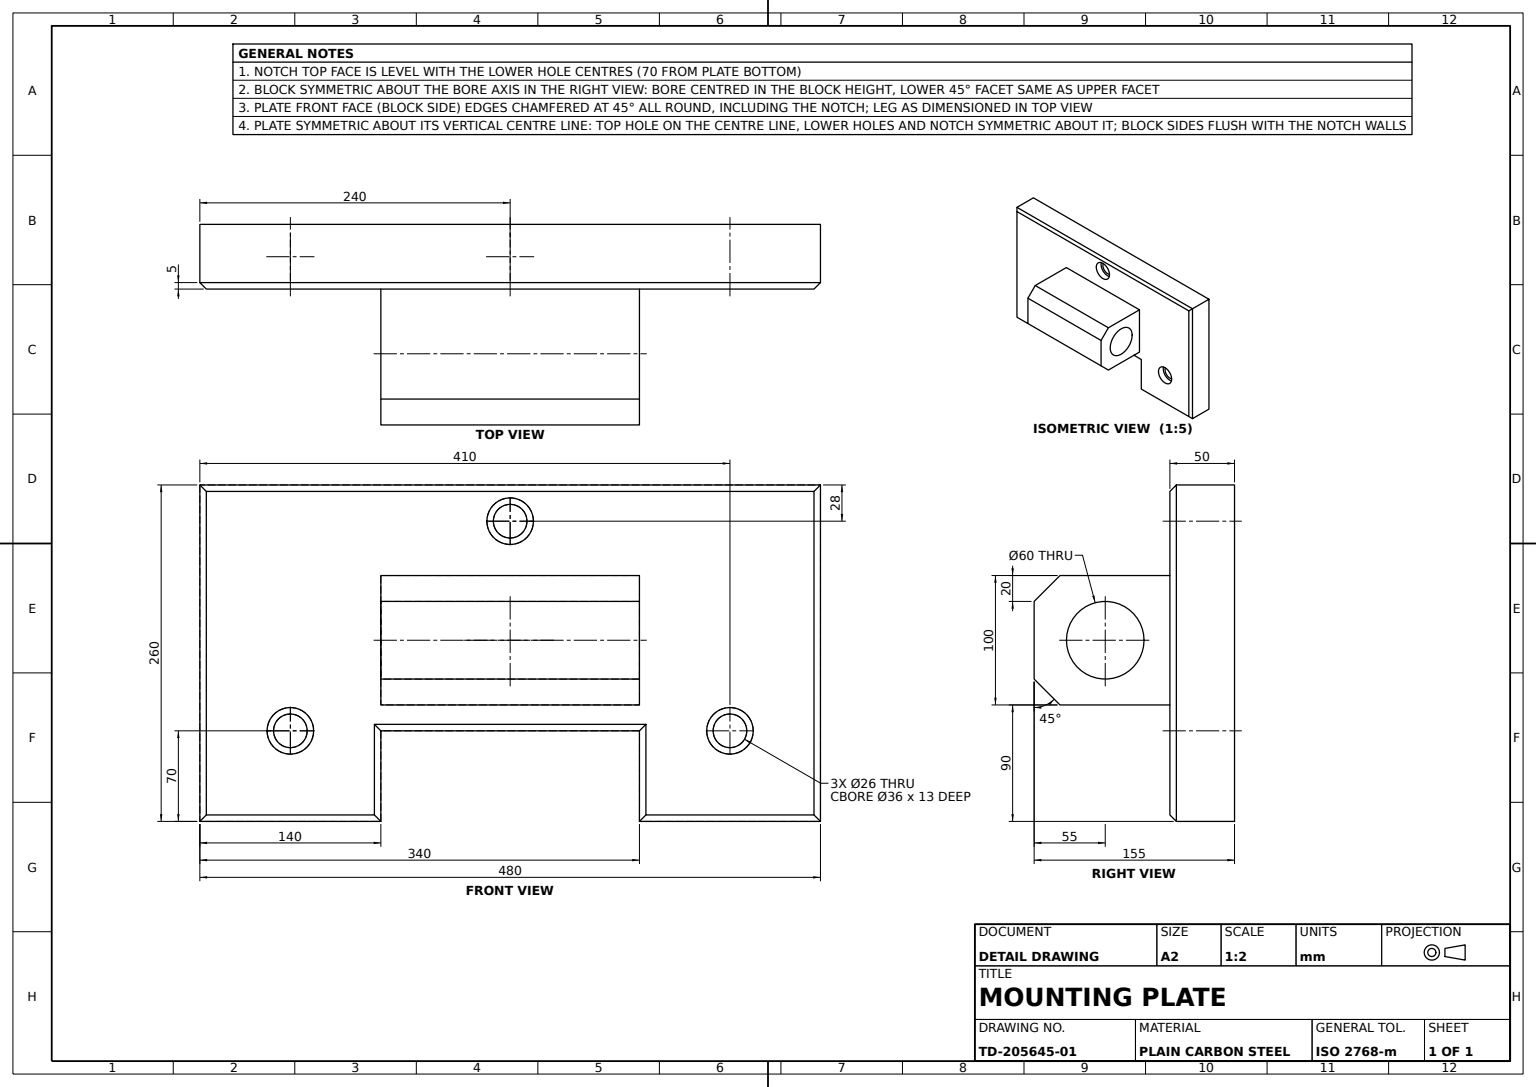
ISO-10303-21;
HEADER;
FILE_DESCRIPTION((''),'2;1');
FILE_NAME('','',(''),(''),'','','');
FILE_SCHEMA(('AUTOMOTIVE_DESIGN'));
ENDSEC;
DATA;
#1=APPLICATION_CONTEXT('');
#2=PRODUCT_CONTEXT('',#1,'mechanical');
#3=PRODUCT('','','',(#2));
#4=PRODUCT_DEFINITION_FORMATION('','',#3);
#5=PRODUCT_DEFINITION_CONTEXT('',#1,'design');
#6=PRODUCT_DEFINITION('','',#4,#5);
#7=PRODUCT_DEFINITION_SHAPE('','',#6);
#8=(LENGTH_UNIT()NAMED_UNIT(*)SI_UNIT(.MILLI.,.METRE.));
#9=(NAMED_UNIT(*)PLANE_ANGLE_UNIT()SI_UNIT($,.RADIAN.));
#10=(NAMED_UNIT(*)SI_UNIT($,.STERADIAN.)SOLID_ANGLE_UNIT());
#11=UNCERTAINTY_MEASURE_WITH_UNIT(LENGTH_MEASURE(1.E-05),#8,'distance_accuracy_value','');
#12=(GEOMETRIC_REPRESENTATION_CONTEXT(3)GLOBAL_UNCERTAINTY_ASSIGNED_CONTEXT((#11))GLOBAL_UNIT_ASSIGNED_CONTEXT((#8,#9,#10))REPRESENTATION_CONTEXT('',''));
#13=CARTESIAN_POINT('',(428.,-190.,37.));
#14=VERTEX_POINT('',#13);
#15=CARTESIAN_POINT('',(428.,-190.,50.));
#16=VERTEX_POINT('',#15);
#17=DIRECTION('',(0.,0.,1.));
#18=VECTOR('',#17,1000.);
#19=LINE('',#13,#18);
#20=EDGE_CURVE('',#14,#16,#19,.T.);
#21=ORIENTED_EDGE('',*,*,#20,.T.);
#22=CARTESIAN_POINT('',(392.,-190.,50.));
#23=VERTEX_POINT('',#22);
#24=CARTESIAN_POINT('',(410.,-190.,50.));
#25=DIRECTION('',(1.,0.,0.));
#26=AXIS2_PLACEMENT_3D('',#24,#17,#25);
#27=CIRCLE('',#26,18.);
#28=EDGE_CURVE('',#16,#23,#27,.T.);
#29=ORIENTED_EDGE('',*,*,#28,.T.);
#30=CARTESIAN_POINT('',(392.,-190.,37.));
#31=VERTEX_POINT('',#30);
#32=LINE('',#30,#18);
#33=EDGE_CURVE('',#31,#23,#32,.T.);
#34=ORIENTED_EDGE('',*,*,#33,.F.);
#35=CARTESIAN_POINT('',(410.,-190.,37.));
#36=AXIS2_PLACEMENT_3D('',#35,#17,#25);
#37=CIRCLE('',#36,18.);
#38=EDGE_CURVE('',#14,#31,#37,.T.);
#39=ORIENTED_EDGE('',*,*,#38,.F.);
#40=EDGE_LOOP('',(#21,#29,#34,#39));
#41=FACE_OUTER_BOUND('',#40,.T.);
#42=CYLINDRICAL_SURFACE('',#36,18.);
#43=ADVANCED_FACE('',(#41),#42,.F.);
#44=CARTESIAN_POINT('',(0.,-260.,45.));
#45=VERTEX_POINT('',#44);
#46=CARTESIAN_POINT('',(5.,-255.,50.));
#47=VERTEX_POINT('',#46);
#48=CARTESIAN_POINT('',(90.,-170.,135.));
#49=DIRECTION('',(0.577350269,0.577350269,0.577350269));
#50=VECTOR('',#49,1000.);
#51=LINE('',#48,#50);
#52=EDGE_CURVE('',#45,#47,#51,.T.);
#53=ORIENTED_EDGE('',*,*,#52,.F.);
#54=CARTESIAN_POINT('',(140.,-260.,45.));
#55=VERTEX_POINT('',#54);
#56=DIRECTION('',(-1.,0.,0.));
#57=VECTOR('',#56,1000.);
#58=LINE('',#54,#57);
#59=EDGE_CURVE('',#55,#45,#58,.T.);
#60=ORIENTED_EDGE('',*,*,#59,.F.);
#61=CARTESIAN_POINT('',(135.,-255.,50.));
#62=VERTEX_POINT('',#61);
#63=CARTESIAN_POINT('',(90.,-210.,95.));
#64=DIRECTION('',(-0.577350269,0.577350269,0.577350269));
#65=VECTOR('',#64,1000.);
#66=LINE('',#63,#65);
#67=EDGE_CURVE('',#55,#62,#66,.T.);
#68=ORIENTED_EDGE('',*,*,#67,.T.);
#69=CARTESIAN_POINT('',(0.,-255.,50.));
#70=VECTOR('',#25,1000.);
#71=LINE('',#69,#70);
#72=EDGE_CURVE('',#47,#62,#71,.T.);
#73=ORIENTED_EDGE('',*,*,#72,.F.);
#74=EDGE_LOOP('',(#53,#60,#68,#73));
#75=FACE_OUTER_BOUND('',#74,.T.);
#76=DIRECTION('',(0.,0.707106781,-0.707106781));
#77=AXIS2_PLACEMENT_3D('',#69,#76,#25);
#78=PLANE('',#77);
#79=ADVANCED_FACE('',(#75),#78,.F.);
#80=CARTESIAN_POINT('',(340.,-90.,155.));
#81=VERTEX_POINT('',#80);
#82=CARTESIAN_POINT('',(140.,-90.,155.));
#83=VERTEX_POINT('',#82);
#84=LINE('',#80,#57);
#85=EDGE_CURVE('',#81,#83,#84,.T.);
#86=ORIENTED_EDGE('',*,*,#85,.F.);
#87=CARTESIAN_POINT('',(340.,-70.,135.));
#88=VERTEX_POINT('',#87);
#89=VECTOR('',#76,1000.);
#90=LINE('',#80,#89);
#91=EDGE_CURVE('',#81,#88,#90,.T.);
#92=ORIENTED_EDGE('',*,*,#91,.T.);
#93=CARTESIAN_POINT('',(140.,-70.,135.));
#94=VERTEX_POINT('',#93);
#95=LINE('',#87,#70);
#96=EDGE_CURVE('',#94,#88,#95,.T.);
#97=ORIENTED_EDGE('',*,*,#96,.F.);
#98=LINE('',#82,#89);
#99=EDGE_CURVE('',#83,#94,#98,.T.);
#100=ORIENTED_EDGE('',*,*,#99,.F.);
#101=EDGE_LOOP('',(#86,#92,#97,#100));
#102=FACE_OUTER_BOUND('',#101,.T.);
#103=DIRECTION('',(0.,0.707106781,0.707106781));
#104=DIRECTION('',(0.,-0.707106781,0.707106781));
#105=AXIS2_PLACEMENT_3D('',#80,#103,#104);
#106=PLANE('',#105);
#107=ADVANCED_FACE('',(#102),#106,.T.);
#108=CARTESIAN_POINT('',(57.,-190.,0.));
#109=VERTEX_POINT('',#108);
#110=CARTESIAN_POINT('',(57.,-190.,37.));
#111=VERTEX_POINT('',#110);
#112=CARTESIAN_POINT('',(57.,-190.,-19.));
#113=LINE('',#112,#18);
#114=EDGE_CURVE('',#109,#111,#113,.T.);
#115=ORIENTED_EDGE('',*,*,#114,.F.);
#116=CARTESIAN_POINT('',(83.,-190.,0.));
#117=VERTEX_POINT('',#116);
#118=CARTESIAN_POINT('',(70.,-190.,0.));
#119=DIRECTION('',(0.,0.,-1.));
#120=AXIS2_PLACEMENT_3D('',#118,#119,#56);
#121=CIRCLE('',#120,13.);
#122=EDGE_CURVE('',#109,#117,#121,.T.);
#123=ORIENTED_EDGE('',*,*,#122,.T.);
#124=CARTESIAN_POINT('',(83.,-190.,37.));
#125=VERTEX_POINT('',#124);
#126=CARTESIAN_POINT('',(83.,-190.,-19.));
#127=LINE('',#126,#18);
#128=EDGE_CURVE('',#117,#125,#127,.T.);
#129=ORIENTED_EDGE('',*,*,#128,.T.);
#130=CARTESIAN_POINT('',(70.,-190.,37.));
#131=AXIS2_PLACEMENT_3D('',#130,#17,#25);
#132=CIRCLE('',#131,13.);
#133=EDGE_CURVE('',#125,#111,#132,.T.);
#134=ORIENTED_EDGE('',*,*,#133,.T.);
#135=EDGE_LOOP('',(#115,#123,#129,#134));
#136=FACE_OUTER_BOUND('',#135,.T.);
#137=CARTESIAN_POINT('',(70.,-190.,-19.));
#138=AXIS2_PLACEMENT_3D('',#137,#17,#25);
#139=CYLINDRICAL_SURFACE('',#138,13.);
#140=ADVANCED_FACE('',(#136),#139,.F.);
#141=CARTESIAN_POINT('',(140.,-120.,70.));
#142=VERTEX_POINT('',#141);
#143=CARTESIAN_POINT('',(140.,-120.,130.));
#144=VERTEX_POINT('',#143);
#145=CARTESIAN_POINT('',(140.,-120.,100.));
#146=AXIS2_PLACEMENT_3D('',#145,#56,#17);
#147=CIRCLE('',#146,30.);
#148=EDGE_CURVE('',#142,#144,#147,.T.);
#149=ORIENTED_EDGE('',*,*,#148,.F.);
#150=EDGE_CURVE('',#144,#142,#147,.T.);
#151=ORIENTED_EDGE('',*,*,#150,.F.);
#152=EDGE_LOOP('',(#149,#151));
#153=FACE_BOUND('',#152,.T.);
#154=CARTESIAN_POINT('',(140.,-170.,135.));
#155=VERTEX_POINT('',#154);
#156=CARTESIAN_POINT('',(140.,-150.,155.));
#157=VERTEX_POINT('',#156);
#158=VECTOR('',#103,1000.);
#159=LINE('',#156,#158);
#160=EDGE_CURVE('',#155,#157,#159,.T.);
#161=ORIENTED_EDGE('',*,*,#160,.T.);
#162=DIRECTION('',(0.,1.,0.));
#163=VECTOR('',#162,1000.);
#164=LINE('',#156,#163);
#165=EDGE_CURVE('',#157,#83,#164,.T.);
#166=ORIENTED_EDGE('',*,*,#165,.T.);
#167=ORIENTED_EDGE('',*,*,#99,.T.);
#168=CARTESIAN_POINT('',(140.,-70.,50.));
#169=VERTEX_POINT('',#168);
#170=LINE('',#93,#18);
#171=EDGE_CURVE('',#169,#94,#170,.T.);
#172=ORIENTED_EDGE('',*,*,#171,.F.);
#173=CARTESIAN_POINT('',(140.,-170.,50.));
#174=VERTEX_POINT('',#173);
#175=CARTESIAN_POINT('',(140.,0.,50.));
#176=LINE('',#175,#163);
#177=EDGE_CURVE('',#174,#169,#176,.T.);
#178=ORIENTED_EDGE('',*,*,#177,.F.);
#179=VECTOR('',#119,1000.);
#180=LINE('',#173,#179);
#181=EDGE_CURVE('',#155,#174,#180,.T.);
#182=ORIENTED_EDGE('',*,*,#181,.F.);
#183=EDGE_LOOP('',(#161,#166,#167,#172,#178,#182));
#184=FACE_OUTER_BOUND('',#183,.T.);
#185=CARTESIAN_POINT('',(140.,0.,170.));
#186=AXIS2_PLACEMENT_3D('',#185,#56,#17);
#187=PLANE('',#186);
#188=ADVANCED_FACE('',(#153,#184),#187,.T.);
#189=CARTESIAN_POINT('',(475.,-255.,50.));
#190=VERTEX_POINT('',#189);
#191=CARTESIAN_POINT('',(480.,-260.,45.));
#192=VERTEX_POINT('',#191);
#193=CARTESIAN_POINT('',(390.,-170.,135.));
#194=DIRECTION('',(0.577350269,-0.577350269,-0.577350269));
#195=VECTOR('',#194,1000.);
#196=LINE('',#193,#195);
#197=EDGE_CURVE('',#190,#192,#196,.T.);
#198=ORIENTED_EDGE('',*,*,#197,.T.);
#199=CARTESIAN_POINT('',(480.,0.,45.));
#200=VERTEX_POINT('',#199);
#201=DIRECTION('',(0.,-1.,0.));
#202=VECTOR('',#201,1000.);
#203=LINE('',#199,#202);
#204=EDGE_CURVE('',#200,#192,#203,.T.);
#205=ORIENTED_EDGE('',*,*,#204,.F.);
#206=CARTESIAN_POINT('',(475.,-5.,50.));
#207=VERTEX_POINT('',#206);
#208=CARTESIAN_POINT('',(316.666667,-163.333333,208.333333));
#209=DIRECTION('',(0.577350269,0.577350269,-0.577350269));
#210=VECTOR('',#209,1000.);
#211=LINE('',#208,#210);
#212=EDGE_CURVE('',#207,#200,#211,.T.);
#213=ORIENTED_EDGE('',*,*,#212,.F.);
#214=CARTESIAN_POINT('',(475.,0.,50.));
#215=LINE('',#214,#163);
#216=EDGE_CURVE('',#190,#207,#215,.T.);
#217=ORIENTED_EDGE('',*,*,#216,.F.);
#218=EDGE_LOOP('',(#198,#205,#213,#217));
#219=FACE_OUTER_BOUND('',#218,.T.);
#220=DIRECTION('',(-0.707106781,0.,-0.707106781));
#221=AXIS2_PLACEMENT_3D('',#214,#220,#162);
#222=PLANE('',#221);
#223=ADVANCED_FACE('',(#219),#222,.F.);
#224=CARTESIAN_POINT('',(140.,-190.,45.));
#225=VERTEX_POINT('',#224);
#226=CARTESIAN_POINT('',(140.,-190.,0.));
#227=VERTEX_POINT('',#226);
#228=CARTESIAN_POINT('',(140.,-190.,50.));
#229=LINE('',#228,#179);
#230=EDGE_CURVE('',#225,#227,#229,.T.);
#231=ORIENTED_EDGE('',*,*,#230,.F.);
#232=LINE('',#224,#202);
#233=EDGE_CURVE('',#225,#55,#232,.T.);
#234=ORIENTED_EDGE('',*,*,#233,.T.);
#235=CARTESIAN_POINT('',(140.,-260.,0.));
#236=VERTEX_POINT('',#235);
#237=CARTESIAN_POINT('',(140.,-260.,50.));
#238=LINE('',#237,#179);
#239=EDGE_CURVE('',#55,#236,#238,.T.);
#240=ORIENTED_EDGE('',*,*,#239,.T.);
#241=LINE('',#226,#163);
#242=EDGE_CURVE('',#236,#227,#241,.T.);
#243=ORIENTED_EDGE('',*,*,#242,.T.);
#244=EDGE_LOOP('',(#231,#234,#240,#243));
#245=FACE_OUTER_BOUND('',#244,.T.);
#246=AXIS2_PLACEMENT_3D('',#228,#56,#17);
#247=PLANE('',#246);
#248=ADVANCED_FACE('',(#245),#247,.F.);
#249=ORIENTED_EDGE('',*,*,#160,.F.);
#250=CARTESIAN_POINT('',(340.,-170.,135.));
#251=VERTEX_POINT('',#250);
#252=LINE('',#154,#57);
#253=EDGE_CURVE('',#251,#155,#252,.T.);
#254=ORIENTED_EDGE('',*,*,#253,.F.);
#255=CARTESIAN_POINT('',(340.,-150.,155.));
#256=VERTEX_POINT('',#255);
#257=LINE('',#255,#158);
#258=EDGE_CURVE('',#251,#256,#257,.T.);
#259=ORIENTED_EDGE('',*,*,#258,.T.);
#260=LINE('',#255,#57);
#261=EDGE_CURVE('',#256,#157,#260,.T.);
#262=ORIENTED_EDGE('',*,*,#261,.T.);
#263=EDGE_LOOP('',(#249,#254,#259,#262));
#264=FACE_OUTER_BOUND('',#263,.T.);
#265=DIRECTION('',(0.,-0.707106781,-0.707106781));
#266=AXIS2_PLACEMENT_3D('',#255,#104,#265);
#267=PLANE('',#266);
#268=ADVANCED_FACE('',(#264),#267,.T.);
#269=CARTESIAN_POINT('',(52.,-190.,50.));
#270=VERTEX_POINT('',#269);
#271=CARTESIAN_POINT('',(88.,-190.,50.));
#272=VERTEX_POINT('',#271);
#273=CARTESIAN_POINT('',(70.,-190.,50.));
#274=AXIS2_PLACEMENT_3D('',#273,#17,#25);
#275=CIRCLE('',#274,18.);
#276=EDGE_CURVE('',#270,#272,#275,.T.);
#277=ORIENTED_EDGE('',*,*,#276,.T.);
#278=CARTESIAN_POINT('',(88.,-190.,37.));
#279=VERTEX_POINT('',#278);
#280=LINE('',#278,#18);
#281=EDGE_CURVE('',#279,#272,#280,.T.);
#282=ORIENTED_EDGE('',*,*,#281,.F.);
#283=CARTESIAN_POINT('',(52.,-190.,37.));
#284=VERTEX_POINT('',#283);
#285=CIRCLE('',#131,18.);
#286=EDGE_CURVE('',#284,#279,#285,.T.);
#287=ORIENTED_EDGE('',*,*,#286,.F.);
#288=LINE('',#283,#18);
#289=EDGE_CURVE('',#284,#270,#288,.T.);
#290=ORIENTED_EDGE('',*,*,#289,.T.);
#291=EDGE_LOOP('',(#277,#282,#287,#290));
#292=FACE_OUTER_BOUND('',#291,.T.);
#293=CYLINDRICAL_SURFACE('',#131,18.);
#294=ADVANCED_FACE('',(#292),#293,.F.);
#295=ORIENTED_EDGE('',*,*,#52,.T.);
#296=CARTESIAN_POINT('',(5.,-5.,50.));
#297=VERTEX_POINT('',#296);
#298=CARTESIAN_POINT('',(5.,0.,50.));
#299=LINE('',#298,#202);
#300=EDGE_CURVE('',#297,#47,#299,.T.);
#301=ORIENTED_EDGE('',*,*,#300,.F.);
#302=CARTESIAN_POINT('',(0.,0.,45.));
#303=VERTEX_POINT('',#302);
#304=CARTESIAN_POINT('',(3.333333,-3.333333,48.333333));
#305=DIRECTION('',(0.577350269,-0.577350269,0.577350269));
#306=VECTOR('',#305,1000.);
#307=LINE('',#304,#306);
#308=EDGE_CURVE('',#303,#297,#307,.T.);
#309=ORIENTED_EDGE('',*,*,#308,.F.);
#310=LINE('',#44,#163);
#311=EDGE_CURVE('',#45,#303,#310,.T.);
#312=ORIENTED_EDGE('',*,*,#311,.F.);
#313=EDGE_LOOP('',(#295,#301,#309,#312));
#314=FACE_OUTER_BOUND('',#313,.T.);
#315=DIRECTION('',(0.707106781,0.,-0.707106781));
#316=AXIS2_PLACEMENT_3D('',#298,#315,#201);
#317=PLANE('',#316);
#318=ADVANCED_FACE('',(#314),#317,.F.);
#319=ORIENTED_EDGE('',*,*,#233,.F.);
#320=CARTESIAN_POINT('',(135.,-185.,50.));
#321=VERTEX_POINT('',#320);
#322=CARTESIAN_POINT('',(73.333333,-123.333333,111.666667));
#323=LINE('',#322,#195);
#324=EDGE_CURVE('',#321,#225,#323,.T.);
#325=ORIENTED_EDGE('',*,*,#324,.F.);
#326=CARTESIAN_POINT('',(135.,0.,50.));
#327=LINE('',#326,#163);
#328=EDGE_CURVE('',#62,#321,#327,.T.);
#329=ORIENTED_EDGE('',*,*,#328,.F.);
#330=ORIENTED_EDGE('',*,*,#67,.F.);
#331=EDGE_LOOP('',(#319,#325,#329,#330));
#332=FACE_OUTER_BOUND('',#331,.T.);
#333=AXIS2_PLACEMENT_3D('',#326,#220,#162);
#334=PLANE('',#333);
#335=ADVANCED_FACE('',(#332),#334,.F.);
#336=CARTESIAN_POINT('',(397.,-190.,37.));
#337=VERTEX_POINT('',#336);
#338=CARTESIAN_POINT('',(423.,-190.,37.));
#339=VERTEX_POINT('',#338);
#340=CIRCLE('',#36,13.);
#341=EDGE_CURVE('',#337,#339,#340,.T.);
#342=ORIENTED_EDGE('',*,*,#341,.F.);
#343=EDGE_CURVE('',#339,#337,#340,.T.);
#344=ORIENTED_EDGE('',*,*,#343,.F.);
#345=EDGE_LOOP('',(#342,#344));
#346=FACE_BOUND('',#345,.T.);
#347=ORIENTED_EDGE('',*,*,#38,.T.);
#348=EDGE_CURVE('',#31,#14,#37,.T.);
#349=ORIENTED_EDGE('',*,*,#348,.T.);
#350=EDGE_LOOP('',(#347,#349));
#351=FACE_OUTER_BOUND('',#350,.T.);
#352=PLANE('',#36);
#353=ADVANCED_FACE('',(#346,#351),#352,.T.);
#354=CARTESIAN_POINT('',(258.,-28.,37.));
#355=VERTEX_POINT('',#354);
#356=CARTESIAN_POINT('',(222.,-28.,37.));
#357=VERTEX_POINT('',#356);
#358=CARTESIAN_POINT('',(240.,-28.,37.));
#359=AXIS2_PLACEMENT_3D('',#358,#17,#25);
#360=CIRCLE('',#359,18.);
#361=EDGE_CURVE('',#355,#357,#360,.T.);
#362=ORIENTED_EDGE('',*,*,#361,.T.);
#363=EDGE_CURVE('',#357,#355,#360,.T.);
#364=ORIENTED_EDGE('',*,*,#363,.T.);
#365=EDGE_LOOP('',(#362,#364));
#366=FACE_OUTER_BOUND('',#365,.T.);
#367=CARTESIAN_POINT('',(253.,-28.,37.));
#368=VERTEX_POINT('',#367);
#369=CARTESIAN_POINT('',(227.,-28.,37.));
#370=VERTEX_POINT('',#369);
#371=CIRCLE('',#359,13.);
#372=EDGE_CURVE('',#368,#370,#371,.T.);
#373=ORIENTED_EDGE('',*,*,#372,.F.);
#374=EDGE_CURVE('',#370,#368,#371,.T.);
#375=ORIENTED_EDGE('',*,*,#374,.F.);
#376=EDGE_LOOP('',(#373,#375));
#377=FACE_BOUND('',#376,.T.);
#378=PLANE('',#359);
#379=ADVANCED_FACE('',(#366,#377),#378,.T.);
#380=EDGE_CURVE('',#279,#284,#285,.T.);
#381=ORIENTED_EDGE('',*,*,#380,.F.);
#382=ORIENTED_EDGE('',*,*,#281,.T.);
#383=EDGE_CURVE('',#272,#270,#275,.T.);
#384=ORIENTED_EDGE('',*,*,#383,.T.);
#385=ORIENTED_EDGE('',*,*,#289,.F.);
#386=EDGE_LOOP('',(#381,#382,#384,#385));
#387=FACE_OUTER_BOUND('',#386,.T.);
#388=ADVANCED_FACE('',(#387),#293,.F.);
#389=EDGE_CURVE('',#23,#16,#27,.T.);
#390=ORIENTED_EDGE('',*,*,#389,.T.);
#391=ORIENTED_EDGE('',*,*,#20,.F.);
#392=ORIENTED_EDGE('',*,*,#348,.F.);
#393=ORIENTED_EDGE('',*,*,#33,.T.);
#394=EDGE_LOOP('',(#390,#391,#392,#393));
#395=FACE_OUTER_BOUND('',#394,.T.);
#396=ADVANCED_FACE('',(#395),#42,.F.);
#397=CARTESIAN_POINT('',(397.,-190.,0.));
#398=VERTEX_POINT('',#397);
#399=CARTESIAN_POINT('',(397.,-190.,-19.));
#400=LINE('',#399,#18);
#401=EDGE_CURVE('',#398,#337,#400,.T.);
#402=ORIENTED_EDGE('',*,*,#401,.F.);
#403=CARTESIAN_POINT('',(423.,-190.,0.));
#404=VERTEX_POINT('',#403);
#405=CARTESIAN_POINT('',(410.,-190.,0.));
#406=AXIS2_PLACEMENT_3D('',#405,#119,#56);
#407=CIRCLE('',#406,13.);
#408=EDGE_CURVE('',#398,#404,#407,.T.);
#409=ORIENTED_EDGE('',*,*,#408,.T.);
#410=CARTESIAN_POINT('',(423.,-190.,-19.));
#411=LINE('',#410,#18);
#412=EDGE_CURVE('',#404,#339,#411,.T.);
#413=ORIENTED_EDGE('',*,*,#412,.T.);
#414=ORIENTED_EDGE('',*,*,#343,.T.);
#415=EDGE_LOOP('',(#402,#409,#413,#414));
#416=FACE_OUTER_BOUND('',#415,.T.);
#417=CARTESIAN_POINT('',(410.,-190.,-19.));
#418=AXIS2_PLACEMENT_3D('',#417,#17,#25);
#419=CYLINDRICAL_SURFACE('',#418,13.);
#420=ADVANCED_FACE('',(#416),#419,.F.);
#421=CARTESIAN_POINT('',(222.,-28.,50.));
#422=VERTEX_POINT('',#421);
#423=LINE('',#356,#18);
#424=EDGE_CURVE('',#357,#422,#423,.T.);
#425=ORIENTED_EDGE('',*,*,#424,.F.);
#426=ORIENTED_EDGE('',*,*,#361,.F.);
#427=CARTESIAN_POINT('',(258.,-28.,50.));
#428=VERTEX_POINT('',#427);
#429=LINE('',#354,#18);
#430=EDGE_CURVE('',#355,#428,#429,.T.);
#431=ORIENTED_EDGE('',*,*,#430,.T.);
#432=CARTESIAN_POINT('',(240.,-28.,50.));
#433=AXIS2_PLACEMENT_3D('',#432,#17,#25);
#434=CIRCLE('',#433,18.);
#435=EDGE_CURVE('',#428,#422,#434,.T.);
#436=ORIENTED_EDGE('',*,*,#435,.T.);
#437=EDGE_LOOP('',(#425,#426,#431,#436));
#438=FACE_OUTER_BOUND('',#437,.T.);
#439=CYLINDRICAL_SURFACE('',#359,18.);
#440=ADVANCED_FACE('',(#438),#439,.F.);
#441=ORIENTED_EDGE('',*,*,#372,.T.);
#442=CARTESIAN_POINT('',(227.,-28.,0.));
#443=VERTEX_POINT('',#442);
#444=CARTESIAN_POINT('',(227.,-28.,-19.));
#445=LINE('',#444,#18);
#446=EDGE_CURVE('',#443,#370,#445,.T.);
#447=ORIENTED_EDGE('',*,*,#446,.F.);
#448=CARTESIAN_POINT('',(253.,-28.,0.));
#449=VERTEX_POINT('',#448);
#450=CARTESIAN_POINT('',(240.,-28.,0.));
#451=AXIS2_PLACEMENT_3D('',#450,#119,#56);
#452=CIRCLE('',#451,13.);
#453=EDGE_CURVE('',#443,#449,#452,.T.);
#454=ORIENTED_EDGE('',*,*,#453,.T.);
#455=CARTESIAN_POINT('',(253.,-28.,-19.));
#456=LINE('',#455,#18);
#457=EDGE_CURVE('',#449,#368,#456,.T.);
#458=ORIENTED_EDGE('',*,*,#457,.T.);
#459=EDGE_LOOP('',(#441,#447,#454,#458));
#460=FACE_OUTER_BOUND('',#459,.T.);
#461=CARTESIAN_POINT('',(240.,-28.,-19.));
#462=AXIS2_PLACEMENT_3D('',#461,#17,#25);
#463=CYLINDRICAL_SURFACE('',#462,13.);
#464=ADVANCED_FACE('',(#460),#463,.F.);
#465=ORIENTED_EDGE('',*,*,#308,.T.);
#466=CARTESIAN_POINT('',(0.,-5.,50.));
#467=LINE('',#466,#57);
#468=EDGE_CURVE('',#207,#297,#467,.T.);
#469=ORIENTED_EDGE('',*,*,#468,.F.);
#470=ORIENTED_EDGE('',*,*,#212,.T.);
#471=LINE('',#302,#70);
#472=EDGE_CURVE('',#303,#200,#471,.T.);
#473=ORIENTED_EDGE('',*,*,#472,.F.);
#474=EDGE_LOOP('',(#465,#469,#470,#473));
#475=FACE_OUTER_BOUND('',#474,.T.);
#476=AXIS2_PLACEMENT_3D('',#466,#265,#56);
#477=PLANE('',#476);
#478=ADVANCED_FACE('',(#475),#477,.F.);
#479=CARTESIAN_POINT('',(340.,-190.,45.));
#480=VERTEX_POINT('',#479);
#481=CARTESIAN_POINT('',(345.,-185.,50.));
#482=VERTEX_POINT('',#481);
#483=CARTESIAN_POINT('',(406.666667,-123.333333,111.666667));
#484=LINE('',#483,#50);
#485=EDGE_CURVE('',#480,#482,#484,.T.);
#486=ORIENTED_EDGE('',*,*,#485,.T.);
#487=CARTESIAN_POINT('',(0.,-185.,50.));
#488=LINE('',#487,#70);
#489=EDGE_CURVE('',#321,#482,#488,.T.);
#490=ORIENTED_EDGE('',*,*,#489,.F.);
#491=ORIENTED_EDGE('',*,*,#324,.T.);
#492=LINE('',#479,#57);
#493=EDGE_CURVE('',#480,#225,#492,.T.);
#494=ORIENTED_EDGE('',*,*,#493,.F.);
#495=EDGE_LOOP('',(#486,#490,#491,#494));
#496=FACE_OUTER_BOUND('',#495,.T.);
#497=AXIS2_PLACEMENT_3D('',#487,#76,#25);
#498=PLANE('',#497);
#499=ADVANCED_FACE('',(#496),#498,.F.);
#500=CARTESIAN_POINT('',(340.,-70.,50.));
#501=VERTEX_POINT('',#500);
#502=CARTESIAN_POINT('',(340.,-170.,50.));
#503=VERTEX_POINT('',#502);
#504=CARTESIAN_POINT('',(340.,0.,50.));
#505=LINE('',#504,#202);
#506=EDGE_CURVE('',#501,#503,#505,.T.);
#507=ORIENTED_EDGE('',*,*,#506,.F.);
#508=LINE('',#500,#179);
#509=EDGE_CURVE('',#88,#501,#508,.T.);
#510=ORIENTED_EDGE('',*,*,#509,.F.);
#511=ORIENTED_EDGE('',*,*,#91,.F.);
#512=LINE('',#255,#163);
#513=EDGE_CURVE('',#256,#81,#512,.T.);
#514=ORIENTED_EDGE('',*,*,#513,.F.);
#515=ORIENTED_EDGE('',*,*,#258,.F.);
#516=LINE('',#250,#18);
#517=EDGE_CURVE('',#503,#251,#516,.T.);
#518=ORIENTED_EDGE('',*,*,#517,.F.);
#519=EDGE_LOOP('',(#507,#510,#511,#514,#515,#518));
#520=FACE_OUTER_BOUND('',#519,.T.);
#521=CARTESIAN_POINT('',(340.,-120.,70.));
#522=VERTEX_POINT('',#521);
#523=CARTESIAN_POINT('',(340.,-120.,130.));
#524=VERTEX_POINT('',#523);
#525=CARTESIAN_POINT('',(340.,-120.,100.));
#526=AXIS2_PLACEMENT_3D('',#525,#56,#17);
#527=CIRCLE('',#526,30.);
#528=EDGE_CURVE('',#522,#524,#527,.T.);
#529=ORIENTED_EDGE('',*,*,#528,.T.);
#530=EDGE_CURVE('',#524,#522,#527,.T.);
#531=ORIENTED_EDGE('',*,*,#530,.T.);
#532=EDGE_LOOP('',(#529,#531));
#533=FACE_BOUND('',#532,.T.);
#534=CARTESIAN_POINT('',(340.,0.,170.));
#535=AXIS2_PLACEMENT_3D('',#534,#25,#119);
#536=PLANE('',#535);
#537=ADVANCED_FACE('',(#520,#533),#536,.T.);
#538=ORIENTED_EDGE('',*,*,#128,.F.);
#539=EDGE_CURVE('',#117,#109,#121,.T.);
#540=ORIENTED_EDGE('',*,*,#539,.T.);
#541=ORIENTED_EDGE('',*,*,#114,.T.);
#542=EDGE_CURVE('',#111,#125,#132,.T.);
#543=ORIENTED_EDGE('',*,*,#542,.T.);
#544=EDGE_LOOP('',(#538,#540,#541,#543));
#545=FACE_OUTER_BOUND('',#544,.T.);
#546=ADVANCED_FACE('',(#545),#139,.F.);
#547=ORIENTED_EDGE('',*,*,#542,.F.);
#548=ORIENTED_EDGE('',*,*,#133,.F.);
#549=EDGE_LOOP('',(#547,#548));
#550=FACE_BOUND('',#549,.T.);
#551=ORIENTED_EDGE('',*,*,#286,.T.);
#552=ORIENTED_EDGE('',*,*,#380,.T.);
#553=EDGE_LOOP('',(#551,#552));
#554=FACE_OUTER_BOUND('',#553,.T.);
#555=PLANE('',#131);
#556=ADVANCED_FACE('',(#550,#554),#555,.T.);
#557=ORIENTED_EDGE('',*,*,#493,.T.);
#558=ORIENTED_EDGE('',*,*,#230,.T.);
#559=CARTESIAN_POINT('',(340.,-190.,0.));
#560=VERTEX_POINT('',#559);
#561=LINE('',#559,#70);
#562=EDGE_CURVE('',#227,#560,#561,.T.);
#563=ORIENTED_EDGE('',*,*,#562,.T.);
#564=CARTESIAN_POINT('',(340.,-190.,50.));
#565=LINE('',#564,#179);
#566=EDGE_CURVE('',#480,#560,#565,.T.);
#567=ORIENTED_EDGE('',*,*,#566,.F.);
#568=EDGE_LOOP('',(#557,#558,#563,#567));
#569=FACE_OUTER_BOUND('',#568,.T.);
#570=AXIS2_PLACEMENT_3D('',#564,#162,#17);
#571=PLANE('',#570);
#572=ADVANCED_FACE('',(#569),#571,.F.);
#573=LINE('',#521,#57);
#574=EDGE_CURVE('',#522,#142,#573,.T.);
#575=ORIENTED_EDGE('',*,*,#574,.F.);
#576=ORIENTED_EDGE('',*,*,#530,.F.);
#577=LINE('',#523,#57);
#578=EDGE_CURVE('',#524,#144,#577,.T.);
#579=ORIENTED_EDGE('',*,*,#578,.T.);
#580=ORIENTED_EDGE('',*,*,#150,.T.);
#581=EDGE_LOOP('',(#575,#576,#579,#580));
#582=FACE_OUTER_BOUND('',#581,.T.);
#583=CYLINDRICAL_SURFACE('',#526,30.);
#584=ADVANCED_FACE('',(#582),#583,.F.);
#585=CARTESIAN_POINT('',(340.,-260.,45.));
#586=VERTEX_POINT('',#585);
#587=CARTESIAN_POINT('',(345.,-255.,50.));
#588=VERTEX_POINT('',#587);
#589=CARTESIAN_POINT('',(430.,-170.,135.));
#590=LINE('',#589,#50);
#591=EDGE_CURVE('',#586,#588,#590,.T.);
#592=ORIENTED_EDGE('',*,*,#591,.T.);
#593=CARTESIAN_POINT('',(345.,0.,50.));
#594=LINE('',#593,#202);
#595=EDGE_CURVE('',#482,#588,#594,.T.);
#596=ORIENTED_EDGE('',*,*,#595,.F.);
#597=ORIENTED_EDGE('',*,*,#485,.F.);
#598=LINE('',#585,#163);
#599=EDGE_CURVE('',#586,#480,#598,.T.);
#600=ORIENTED_EDGE('',*,*,#599,.F.);
#601=EDGE_LOOP('',(#592,#596,#597,#600));
#602=FACE_OUTER_BOUND('',#601,.T.);
#603=AXIS2_PLACEMENT_3D('',#593,#315,#201);
#604=PLANE('',#603);
#605=ADVANCED_FACE('',(#602),#604,.F.);
#606=ORIENTED_EDGE('',*,*,#122,.F.);
#607=ORIENTED_EDGE('',*,*,#539,.F.);
#608=EDGE_LOOP('',(#606,#607));
#609=FACE_BOUND('',#608,.T.);
#610=ORIENTED_EDGE('',*,*,#562,.F.);
#611=ORIENTED_EDGE('',*,*,#242,.F.);
#612=CARTESIAN_POINT('',(0.,-260.,0.));
#613=VERTEX_POINT('',#612);
#614=LINE('',#235,#70);
#615=EDGE_CURVE('',#613,#236,#614,.T.);
#616=ORIENTED_EDGE('',*,*,#615,.F.);
#617=CARTESIAN_POINT('',(0.,0.,0.));
#618=VERTEX_POINT('',#617);
#619=LINE('',#612,#202);
#620=EDGE_CURVE('',#618,#613,#619,.T.);
#621=ORIENTED_EDGE('',*,*,#620,.F.);
#622=CARTESIAN_POINT('',(480.,0.,0.));
#623=VERTEX_POINT('',#622);
#624=LINE('',#617,#57);
#625=EDGE_CURVE('',#623,#618,#624,.T.);
#626=ORIENTED_EDGE('',*,*,#625,.F.);
#627=CARTESIAN_POINT('',(480.,-260.,0.));
#628=VERTEX_POINT('',#627);
#629=LINE('',#622,#163);
#630=EDGE_CURVE('',#628,#623,#629,.T.);
#631=ORIENTED_EDGE('',*,*,#630,.F.);
#632=CARTESIAN_POINT('',(340.,-260.,0.));
#633=VERTEX_POINT('',#632);
#634=LINE('',#627,#70);
#635=EDGE_CURVE('',#633,#628,#634,.T.);
#636=ORIENTED_EDGE('',*,*,#635,.F.);
#637=LINE('',#632,#202);
#638=EDGE_CURVE('',#560,#633,#637,.T.);
#639=ORIENTED_EDGE('',*,*,#638,.F.);
#640=EDGE_LOOP('',(#610,#611,#616,#621,#626,#631,#636,#639));
#641=FACE_OUTER_BOUND('',#640,.T.);
#642=EDGE_CURVE('',#449,#443,#452,.T.);
#643=ORIENTED_EDGE('',*,*,#642,.F.);
#644=ORIENTED_EDGE('',*,*,#453,.F.);
#645=EDGE_LOOP('',(#643,#644));
#646=FACE_BOUND('',#645,.T.);
#647=EDGE_CURVE('',#404,#398,#407,.T.);
#648=ORIENTED_EDGE('',*,*,#647,.F.);
#649=ORIENTED_EDGE('',*,*,#408,.F.);
#650=EDGE_LOOP('',(#648,#649));
#651=FACE_BOUND('',#650,.T.);
#652=AXIS2_PLACEMENT_3D('',#617,#119,#56);
#653=PLANE('',#652);
#654=ADVANCED_FACE('',(#609,#641,#646,#651),#653,.T.);
#655=ORIENTED_EDGE('',*,*,#513,.T.);
#656=ORIENTED_EDGE('',*,*,#85,.T.);
#657=ORIENTED_EDGE('',*,*,#165,.F.);
#658=ORIENTED_EDGE('',*,*,#261,.F.);
#659=EDGE_LOOP('',(#655,#656,#657,#658));
#660=FACE_OUTER_BOUND('',#659,.T.);
#661=AXIS2_PLACEMENT_3D('',#255,#17,#25);
#662=PLANE('',#661);
#663=ADVANCED_FACE('',(#660),#662,.T.);
#664=ORIENTED_EDGE('',*,*,#171,.T.);
#665=ORIENTED_EDGE('',*,*,#96,.T.);
#666=ORIENTED_EDGE('',*,*,#509,.T.);
#667=LINE('',#168,#57);
#668=EDGE_CURVE('',#501,#169,#667,.T.);
#669=ORIENTED_EDGE('',*,*,#668,.T.);
#670=EDGE_LOOP('',(#664,#665,#666,#669));
#671=FACE_OUTER_BOUND('',#670,.T.);
#672=CARTESIAN_POINT('',(0.,-70.,0.));
#673=AXIS2_PLACEMENT_3D('',#672,#201,#119);
#674=PLANE('',#673);
#675=ADVANCED_FACE('',(#671),#674,.F.);
#676=ORIENTED_EDGE('',*,*,#148,.T.);
#677=ORIENTED_EDGE('',*,*,#578,.F.);
#678=ORIENTED_EDGE('',*,*,#528,.F.);
#679=ORIENTED_EDGE('',*,*,#574,.T.);
#680=EDGE_LOOP('',(#676,#677,#678,#679));
#681=FACE_OUTER_BOUND('',#680,.T.);
#682=ADVANCED_FACE('',(#681),#583,.F.);
#683=ORIENTED_EDGE('',*,*,#620,.T.);
#684=CARTESIAN_POINT('',(0.,-260.,50.));
#685=LINE('',#684,#179);
#686=EDGE_CURVE('',#45,#613,#685,.T.);
#687=ORIENTED_EDGE('',*,*,#686,.F.);
#688=ORIENTED_EDGE('',*,*,#311,.T.);
#689=CARTESIAN_POINT('',(0.,0.,50.));
#690=LINE('',#689,#179);
#691=EDGE_CURVE('',#303,#618,#690,.T.);
#692=ORIENTED_EDGE('',*,*,#691,.T.);
#693=EDGE_LOOP('',(#683,#687,#688,#692));
#694=FACE_OUTER_BOUND('',#693,.T.);
#695=AXIS2_PLACEMENT_3D('',#684,#25,#119);
#696=PLANE('',#695);
#697=ADVANCED_FACE('',(#694),#696,.F.);
#698=ORIENTED_EDGE('',*,*,#28,.F.);
#699=ORIENTED_EDGE('',*,*,#389,.F.);
#700=EDGE_LOOP('',(#698,#699));
#701=FACE_BOUND('',#700,.T.);
#702=EDGE_CURVE('',#422,#428,#434,.T.);
#703=ORIENTED_EDGE('',*,*,#702,.F.);
#704=ORIENTED_EDGE('',*,*,#435,.F.);
#705=EDGE_LOOP('',(#703,#704));
#706=FACE_BOUND('',#705,.T.);
#707=ORIENTED_EDGE('',*,*,#595,.T.);
#708=EDGE_CURVE('',#588,#190,#71,.T.);
#709=ORIENTED_EDGE('',*,*,#708,.T.);
#710=ORIENTED_EDGE('',*,*,#216,.T.);
#711=ORIENTED_EDGE('',*,*,#468,.T.);
#712=ORIENTED_EDGE('',*,*,#300,.T.);
#713=ORIENTED_EDGE('',*,*,#72,.T.);
#714=ORIENTED_EDGE('',*,*,#328,.T.);
#715=ORIENTED_EDGE('',*,*,#489,.T.);
#716=EDGE_LOOP('',(#707,#709,#710,#711,#712,#713,#714,#715));
#717=FACE_OUTER_BOUND('',#716,.T.);
#718=ORIENTED_EDGE('',*,*,#177,.T.);
#719=ORIENTED_EDGE('',*,*,#668,.F.);
#720=ORIENTED_EDGE('',*,*,#506,.T.);
#721=LINE('',#502,#70);
#722=EDGE_CURVE('',#174,#503,#721,.T.);
#723=ORIENTED_EDGE('',*,*,#722,.F.);
#724=EDGE_LOOP('',(#718,#719,#720,#723));
#725=FACE_BOUND('',#724,.T.);
#726=ORIENTED_EDGE('',*,*,#383,.F.);
#727=ORIENTED_EDGE('',*,*,#276,.F.);
#728=EDGE_LOOP('',(#726,#727));
#729=FACE_BOUND('',#728,.T.);
#730=AXIS2_PLACEMENT_3D('',#689,#119,#56);
#731=PLANE('',#730);
#732=ADVANCED_FACE('',(#701,#706,#717,#725,#729),#731,.F.);
#733=ORIENTED_EDGE('',*,*,#647,.T.);
#734=ORIENTED_EDGE('',*,*,#401,.T.);
#735=ORIENTED_EDGE('',*,*,#341,.T.);
#736=ORIENTED_EDGE('',*,*,#412,.F.);
#737=EDGE_LOOP('',(#733,#734,#735,#736));
#738=FACE_OUTER_BOUND('',#737,.T.);
#739=ADVANCED_FACE('',(#738),#419,.F.);
#740=ORIENTED_EDGE('',*,*,#722,.T.);
#741=ORIENTED_EDGE('',*,*,#517,.T.);
#742=ORIENTED_EDGE('',*,*,#253,.T.);
#743=ORIENTED_EDGE('',*,*,#181,.T.);
#744=EDGE_LOOP('',(#740,#741,#742,#743));
#745=FACE_OUTER_BOUND('',#744,.T.);
#746=CARTESIAN_POINT('',(0.,-170.,0.));
#747=AXIS2_PLACEMENT_3D('',#746,#162,#17);
#748=PLANE('',#747);
#749=ADVANCED_FACE('',(#745),#748,.F.);
#750=LINE('',#191,#57);
#751=EDGE_CURVE('',#192,#586,#750,.T.);
#752=ORIENTED_EDGE('',*,*,#751,.T.);
#753=CARTESIAN_POINT('',(340.,-260.,50.));
#754=LINE('',#753,#179);
#755=EDGE_CURVE('',#586,#633,#754,.T.);
#756=ORIENTED_EDGE('',*,*,#755,.T.);
#757=ORIENTED_EDGE('',*,*,#635,.T.);
#758=CARTESIAN_POINT('',(480.,-260.,50.));
#759=LINE('',#758,#179);
#760=EDGE_CURVE('',#192,#628,#759,.T.);
#761=ORIENTED_EDGE('',*,*,#760,.F.);
#762=EDGE_LOOP('',(#752,#756,#757,#761));
#763=FACE_OUTER_BOUND('',#762,.T.);
#764=AXIS2_PLACEMENT_3D('',#758,#162,#17);
#765=PLANE('',#764);
#766=ADVANCED_FACE('',(#763),#765,.F.);
#767=ORIENTED_EDGE('',*,*,#638,.T.);
#768=ORIENTED_EDGE('',*,*,#755,.F.);
#769=ORIENTED_EDGE('',*,*,#599,.T.);
#770=ORIENTED_EDGE('',*,*,#566,.T.);
#771=EDGE_LOOP('',(#767,#768,#769,#770));
#772=FACE_OUTER_BOUND('',#771,.T.);
#773=AXIS2_PLACEMENT_3D('',#753,#25,#119);
#774=PLANE('',#773);
#775=ADVANCED_FACE('',(#772),#774,.F.);
#776=ORIENTED_EDGE('',*,*,#204,.T.);
#777=ORIENTED_EDGE('',*,*,#760,.T.);
#778=ORIENTED_EDGE('',*,*,#630,.T.);
#779=CARTESIAN_POINT('',(480.,0.,50.));
#780=LINE('',#779,#179);
#781=EDGE_CURVE('',#200,#623,#780,.T.);
#782=ORIENTED_EDGE('',*,*,#781,.F.);
#783=EDGE_LOOP('',(#776,#777,#778,#782));
#784=FACE_OUTER_BOUND('',#783,.T.);
#785=AXIS2_PLACEMENT_3D('',#779,#56,#17);
#786=PLANE('',#785);
#787=ADVANCED_FACE('',(#784),#786,.F.);
#788=ORIENTED_EDGE('',*,*,#781,.T.);
#789=ORIENTED_EDGE('',*,*,#625,.T.);
#790=ORIENTED_EDGE('',*,*,#691,.F.);
#791=ORIENTED_EDGE('',*,*,#472,.T.);
#792=EDGE_LOOP('',(#788,#789,#790,#791));
#793=FACE_OUTER_BOUND('',#792,.T.);
#794=AXIS2_PLACEMENT_3D('',#689,#201,#119);
#795=PLANE('',#794);
#796=ADVANCED_FACE('',(#793),#795,.F.);
#797=ORIENTED_EDGE('',*,*,#615,.T.);
#798=ORIENTED_EDGE('',*,*,#239,.F.);
#799=ORIENTED_EDGE('',*,*,#59,.T.);
#800=ORIENTED_EDGE('',*,*,#686,.T.);
#801=EDGE_LOOP('',(#797,#798,#799,#800));
#802=FACE_OUTER_BOUND('',#801,.T.);
#803=AXIS2_PLACEMENT_3D('',#237,#162,#17);
#804=PLANE('',#803);
#805=ADVANCED_FACE('',(#802),#804,.F.);
#806=ORIENTED_EDGE('',*,*,#751,.F.);
#807=ORIENTED_EDGE('',*,*,#197,.F.);
#808=ORIENTED_EDGE('',*,*,#708,.F.);
#809=ORIENTED_EDGE('',*,*,#591,.F.);
#810=EDGE_LOOP('',(#806,#807,#808,#809));
#811=FACE_OUTER_BOUND('',#810,.T.);
#812=ADVANCED_FACE('',(#811),#78,.F.);
#813=ORIENTED_EDGE('',*,*,#363,.F.);
#814=ORIENTED_EDGE('',*,*,#424,.T.);
#815=ORIENTED_EDGE('',*,*,#702,.T.);
#816=ORIENTED_EDGE('',*,*,#430,.F.);
#817=EDGE_LOOP('',(#813,#814,#815,#816));
#818=FACE_OUTER_BOUND('',#817,.T.);
#819=ADVANCED_FACE('',(#818),#439,.F.);
#820=ORIENTED_EDGE('',*,*,#457,.F.);
#821=ORIENTED_EDGE('',*,*,#642,.T.);
#822=ORIENTED_EDGE('',*,*,#446,.T.);
#823=ORIENTED_EDGE('',*,*,#374,.T.);
#824=EDGE_LOOP('',(#820,#821,#822,#823));
#825=FACE_OUTER_BOUND('',#824,.T.);
#826=ADVANCED_FACE('',(#825),#463,.F.);
#827=CLOSED_SHELL('',(#43,#79,#107,#140,#188,#223,#248,#268,#294,#318,#335,#353,#379,#388,#396,#420,#440,#464,#478,#499,#537,#546,#556,#572,#584,#605,#654,#663,#675,#682,#697,#732,#739,#749,#766,#775,#787,#796,#805,#812,#819,#826));
#828=MANIFOLD_SOLID_BREP('',#827);
#829=ADVANCED_BREP_SHAPE_REPRESENTATION('',(#828),#12);
#830=SHAPE_DEFINITION_REPRESENTATION(#7,#829);
ENDSEC;
END-ISO-10303-21;
